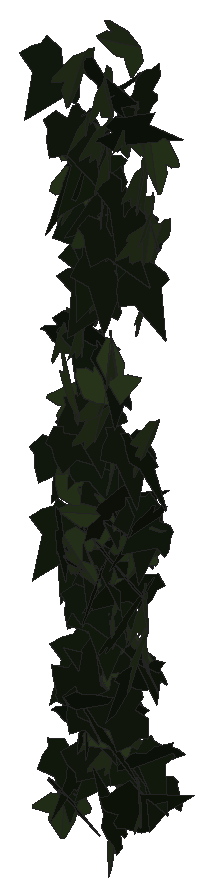
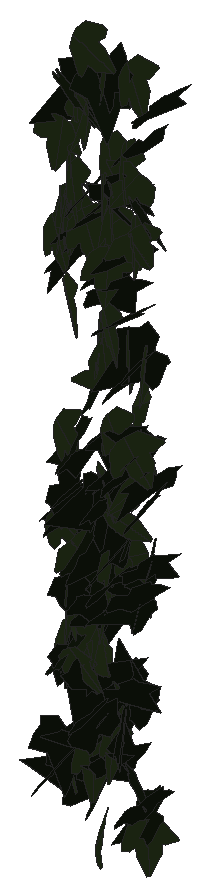
# SketchUp Ruby script. Lengths in inches.
U = 1.inch
M = Sketchup.active_model
def pt(a) = Geom::Point3d.new(a.map { |v| v * U })
def face(e, loops, mat)
  f = e.add_face(loops[0].map { |a| pt(a) })
  loops[1..].each { |l| e.add_face(l.map { |a| pt(a) }).erase! }
  f.material = f.back_material = mat if mat
  f
end
# faces: each face lists its corners as indices into pts; further lists are holes
def faces(e, pts, list, mat = nil) = list.each { |f| face(e, (f[0].is_a?(Array) ? f : [f]).map { |l| l.map { |i| pts[i] } }, mat) }
# xy, xz, yz: faces in a plane at the given z, y or x. An outline is a flat list of corners, or four numbers for a rectangle; further outlines are holes
def ring(l) = l.size == 4 ? [[l[0], l[1]], [l[2], l[1]], [l[2], l[3]], [l[0], l[3]]] : l.each_slice(2).to_a
def flat(e, list, mat, &to3) = list.each { |f| face(e, (f[0].is_a?(Array) ? f : [f]).map { |l| ring(l).map { |u, v| to3.(u, v) } }, mat) }
def xy(e, z, list, mat = nil) = flat(e, list, mat) { |x, y| [x, y, z] }
def xz(e, y, list, mat = nil) = flat(e, list, mat) { |x, z| [x, y, z] }
def yz(e, x, list, mat = nil) = flat(e, list, mat) { |y, z| [x, y, z] }
def lines(e, pts, list) = list.each { |a, b| e.add_line(pt(pts[a]), pt(pts[b])) }
# prism: a flat outline (further loops are holes) pulled along v
def prism(e, loops, v, mat = nil)
  f = face(e, loops, mat); d = Geom::Vector3d.new(v.map { |x| x * U })
  f.pushpull(f.normal.samedirection?(d) ? d.length : -d.length)
end
def box(e, o, s, mat = nil) = prism(e, [[o, [o[0] + s[0], o[1], o[2]], [o[0] + s[0], o[1] + s[1], o[2]], [o[0], o[1] + s[1], o[2]]]], [0, 0, s[2]], mat)
def at(x, y, z, deg = 0) = Geom::Transformation.translation(pt([x, y, z])) * Geom::Transformation.rotation(ORIGIN, Z_AXIS, deg.degrees)
def axes(o, x, y, z) = Geom::Transformation.new([*x, 0, *y, 0, *z, 0, *pt(o).to_a, 1])
def part(name) = M.definitions.add(name)
# library, detail: a bought-in or finely detailed component or shape, given as its bounding box
def library(name, o, s) = part(name).tap { |d| box(d.entities, o, s) }
def detail(e, o, s) = box(e.add_group.entities, o, s)
def put(e, d, t, mat = nil) = e.add_instance(d, t).tap { |i| i.material = mat if mat }
def group(e, t, mat = nil) = e.add_group.tap { |g| g.transformation = t; g.material = mat if mat }.entities
root = M.entities
M.materials.add("efeu1").color = [18, 25, 13]
M.materials.add("efeu2").color = [43, 57, 29]
c1 = part("ivyleaf_9")
p = [[1.54,2.16,1.25],[1.36,2.04,1.19],[-0.21,0.99,0.68],[-0.71,1.11,0.82],[-0.85,0.86,0.67],[-0.8,0.17,0.21],
  [-0.9,-0.01,0.1],[-0.67,-0.16,-0.02],[-0.08,-0.08,-0.05],[-0.03,-0.6,-0.4],[0.65,-0.88,-0.66],[0.83,-0.6,-0.49],
  [1.29,-0.42,-0.43],[1.8125,-0.07,-0.26],[1.21,0.44,0.15]]
faces(c1.entities,p,[[0,1,2,3,4,5,6,7,8,9,10,11,12,13,14]],"efeu1")
c2 = part("ivyleaf_10")
p = [[0,0.5,-0.03],[-0.0625,2.02,-0.43],[-0.19,2.01,-0.46],[-0.54,1.05,-0.29],[-0.52,0.625,-0.18],[-0.83,0.76,-0.28],
  [-1.16,0.64,-0.33],[-1.15,0.33,-0.24],[-0.77,-0.39,0.02],[-0.3,-0.51,0.16],[0.04,-0.48,0.23],[-0.02,2.01,-0.4375],
  [-0.06,2.01,-0.43],[0.04,-0.49,0.23],[0.67,-0.49,0.14],[1.38,0.36,-0.2],[1.375,0.51,-0.24],[0.81,0.65,-0.19],
  [0.62,0.59,-0.15],[0.6,1.09,-0.28],[0.5,1.23,-0.31]]
faces(c2.entities,p,[[0,1,2,3,4,5,6,7,8,9,10],[11,12,0,13,14,15,16,17,18,19,20]],"efeu2")
put(root,c1,axes([542.89,131,239.64],[-0.3779,-0.8089,0.46344],[-0.07293,-0.47288,-0.88486],[0.9294,-0.36601,0.119]))
put(root,c2,axes([543.15,130.99,206.96],[-0.66582,-0.57985,0.08363],[-0.05947,-0.05906,-0.8829],[0.58282,-0.66845,0.00546]))
put(root,c2,axes([543.24,131.94,224.62],[-0.46964,-0.72041,0.42452],[-0.13793,-0.41349,-0.85427],[0.82474,-0.47938,0.09887]))
put(root,c1,axes([542.82,131.93,221.74],[-0.12699,-0.71118,0.61671],[-0.01814,-0.62033,-0.71909],[0.94115,-0.10791,0.06936]))
put(root,c1,axes([543.11,131.42,219.04],[-0.50635,-0.73157,0.28551],[-0.10708,-0.27222,-0.88743],[0.77798,-0.51362,0.06369]))
put(root,c1,axes([542.8,131.78,208.6],[-0.04358,-0.93003,-0.03017],[0.00357,0.03004,-0.93105],[0.93051,-0.04368,0.00216]))
put(root,c2,axes([543.08,131.96,234.19],[0.53623,0.70675,-0.40833],[-0.22326,-0.34294,-0.88675],[-0.78511,0.58024,-0.02673]))
put(root,c1,axes([543.21,130.5625,219.21],[0.54428,-0.26203,-0.88304],[-0.79645,0.38135,-0.60406],[0.46269,0.96466,-0.00106]))
put(root,c1,axes([543.11,132.07,218.12],[-0.41071,-0.80099,0.01291],[-0.00596,-0.01145,-0.90014],[0.80107,-0.41075,-0.00008]))
put(root,c2,axes([543.24,130.78,228.1875],[0.2371,-0.77248,-0.49054],[0.00963,0.50882,-0.79661],[0.91502,0.19481,0.13549]))
put(root,c1,axes([542.89,130.81,222.96],[0.25631,-0.73221,-0.599],[-0.01345,0.61771,-0.76084],[0.94591,0.20718,0.15149]))
put(root,c2,axes([543.45,131.22,234.19],[0.25548,-0.8284,-0.44473],[-0.05712,0.44633,-0.86419],[0.93849,0.25267,0.06846]))
put(root,c1,axes([543.02,130.64,207.7],[0.81346,-0.27877,0.04132],[0.03921,-0.01305,-0.8599],[0.27908,0.8144,0.00037]))
put(root,c1,axes([543.76,131.79,213.49],[-0.66827,-0.54794,0.11511],[-0.07608,-0.08871,-0.86395],[0.5547,-0.67228,0.02018]))
put(root,c1,axes([543.73,131.04,235.24],[-0.79982,0.24945,-0.51189],[0.47089,-0.20653,-0.83641],[-0.32019,-0.92687,0.04861]))
put(root,c2,axes([544.18,130.14,225.47],[-0.27405,0.55462,-0.9475],[-0.55224,0.7744,0.61302],[0.94889,0.61087,0.08313]))
put(root,c1,axes([543.25,130.58,228.39],[0.79583,0.38797,0.34315],[0.32353,0.1189,-0.88476],[-0.40447,0.85846,-0.03254]))
put(root,c1,axes([543.98,130.84,209],[-0.70461,0.24131,-0.4589],[0.41968,-0.18919,-0.74389],[-0.30444,-0.81931,0.03662]))
put(root,c2,axes([543.3,131.49,236.58],[0.75396,0.17984,0.59982],[0.55207,0.25216,-0.76955],[-0.29553,0.92987,0.09268]))
put(root,c1,axes([543.61,131.87,227.56],[-0.02808,-0.90071,0.3593],[0.01235,-0.35976,-0.90088],[0.96965,-0.0215,0.02187]))
put(root,c1,axes([543.73,131.95,223.26],[-0.18829,-0.87979,0.447],[-0.05558,-0.44489,-0.89904],[0.98526,-0.19323,0.03471]))
put(root,c2,axes([543.9375,130.125,222.19],[-0.0737,0.28472,1.03336],[-0.16617,1.02025,-0.29295],[-1.05891,-0.17992,-0.02595]))
put(root,c1,axes([543.26,130.9375,217.57],[0.98692,-0.25548,0.22779],[0.22591,-0.0361,-1.01923],[0.25715,1.01222,0.02114]))
put(root,c2,axes([544.03,131.05,237.25],[0.23393,-0.93139,-0.19948],[0.08891,0.22586,-0.95031],[0.94835,0.20857,0.1383]))
put(root,c2,axes([544.125,130.74,228.55],[0.32713,-0.84864,-0.28411],[0.0021,0.30322,-0.90332],[0.89493,0.3095,0.10597]))
put(root,c1,axes([543.73,130.49,224.01],[0.38574,-0.46473,-0.76294],[-0.14643,0.7869,-0.55336],[0.88126,0.33417,0.24201]))
put(root,c1,axes([543.72,130.51,237.65],[0.33057,-0.8505,-0.42959],[-0.06936,0.43203,-0.90869],[0.95031,0.32738,0.08312]))
put(root,c1,axes([543.9375,131.6,232.93],[-0.14804,-0.95082,-0.18639],[0.03232,0.1836,-0.96227],[0.96838,-0.15148,0.00362]))
put(root,c2,axes([544.27,130.5,240.52],[0.02264,-1.00792,0.16981],[0.02162,-0.16934,-1.00802],[1.0219,0.02591,0.01756]))
put(root,c1,axes([544.13,131.85,229.92],[-0.44896,-0.79228,0.37654],[0.09111,-0.46282,-0.86518],[0.87246,-0.35936,0.28412]))
put(root,c1,axes([543.89,131.62,211.62],[0.0403,-0.11201,-0.9374],[0.79808,-0.49716,0.09371],[-0.50431,-0.79572,0.0734]))
put(root,c2,axes([544.4,131.86,230.02],[0.379,-0.88542,-0.04677],[-0.01625,0.04392,-0.96312],[0.8865,0.37934,0.00234]))
put(root,c1,axes([544.57,131.59,235.91],[-0.80316,-0.57999,0.09291],[-0.08006,-0.04783,-0.99065],[0.5819,-0.8071,-0.00805]))
put(root,c1,axes([544.35,131.87,231.39],[-0.5032,-0.82989,0.02779],[-0.00045,-0.03222,-0.97039],[0.83035,-0.50294,0.01632]))
put(root,c1,axes([544.13,131.45,224.69],[-0.21768,-0.82836,-0.40314],[0.13178,0.38199,-0.85604],[0.91178,-0.25297,0.02747]))
put(root,c1,axes([544.17,132.02,218.18],[-0.14497,-0.949,0.24615],[0.01215,-0.25055,-0.95879],[0.98032,-0.13723,0.04829]))
put(root,c1,axes([543.91,131.52,211.12],[0.14321,-0.23238,-0.90435],[0.84805,-0.35047,0.22435],[-0.39071,-0.84589,0.15549]))
put(root,c2,axes([545.1,130.76,220.5625],[0.31254,0.01615,-0.956],[-0.93757,0.20243,-0.3031],[0.18752,0.98521,0.07795]))
put(root,c2,axes([544.49,131.76,232.7],[-0.53636,-0.82147,-0.06115],[0.08949,0.01443,-0.97878],[0.81887,-0.53964,0.06691]))
put(root,c2,axes([544.5,131.44,225.03],[0.09234,-0.92048,0.18319],[0.01015,-0.18308,-0.92507],[0.93848,0.09255,-0.00802]))
put(root,c1,axes([544.41,130.3,212.39],[-0.74534,0.16412,0.5402],[0.45539,-0.35408,0.73589],[0.33373,0.84969,0.20232]))
put(root,c2,axes([544.63,131.23,210.75],[-0.02239,-0.81588,-0.30481],[0.00737,0.30473,-0.81619],[0.87093,-0.02355,-0.00093]))
put(root,c2,axes([544,130.43,218.94],[-0.51949,0.16153,-0.83821],[0.72315,-0.43811,-0.53261],[-0.45359,-0.88348,0.11086]))
put(root,c2,axes([544.66,131.21,218.7],[-0.08775,-0.87943,-0.25482],[-0.0076,0.25667,-0.88322],[0.91557,-0.08215,-0.03175]))
put(root,c1,axes([544.78,131,209.34],[-0.52719,-0.63291,0.45548],[0.34478,0.30394,0.8214],[-0.6994,0.6269,0.0616]))
put(root,c2,axes([544.75,130.97,224.47],[-0.00558,-0.9292,-0.11369],[-0.03149,0.11381,-0.92867],[0.9356,-0.00171,-0.03193]))
put(root,c1,axes([544.39,131.28,222.88],[0.14621,-0.82186,-0.40667],[0.00957,0.41315,-0.83152],[0.91692,0.12674,0.07352]))
put(root,c2,axes([544.85,131.14,237.3125],[0.13517,-0.99131,-0.1389],[-0.00715,0.1392,-1.00042],[1.00097,0.13486,0.01161]))
put(root,c1,axes([544.45,130.69,212.2],[0.36629,-0.81594,-0.43061],[-0.13641,0.41031,-0.89352],[0.91245,0.38889,0.03928]))
put(root,c1,axes([544.77,132.06,217.47],[-0.32741,-0.90946,-0.21573],[0.04375,0.21342,-0.96612],[0.93367,-0.32892,-0.03038]))
put(root,c1,axes([545.21,131.78,209.6],[-0.64334,-0.61132,0.22429],[-0.1528,-0.16477,-0.88736],[0.63298,-0.6611,0.01376]))
put(root,c1,axes([544.54,129.71,212.3],[0.83497,0.39922,0.37226],[0.32663,0.17967,-0.92529],[-0.43735,0.89637,0.01967]))
put(root,c1,axes([544.62,131.47,218.85],[0.33232,-0.87598,-0.00707],[-0.00069,0.0073,-0.9369],[0.87601,0.33232,0.00195]))
put(root,c2,axes([545.07,131.38,222.36],[0.624,-0.68664,0.00438],[-0.00723,-0.01249,-0.92772],[0.68661,0.62389,-0.01375]))
put(root,c2,axes([545.13,131.06,236.22],[0.3469,-0.84828,-0.3577],[0.02301,0.39012,-0.90286],[0.92033,0.31,0.1574]))
put(root,c1,axes([544.77,131.49,221.6],[0.17194,-0.89909,-0.13673],[-0.04854,0.12988,-0.91509],[0.90813,0.17717,-0.02302]))
put(root,c1,axes([545.71,131.39,212.71],[0.01896,0.05867,0.96721],[-0.96899,0.00306,0.01881],[-0.00192,-0.96739,0.05871]))
put(root,c2,axes([545.12,130.93,234.16],[-0.39132,0.84013,-0.29287],[-0.08317,-0.35309,-0.90174],[-0.88582,-0.33799,0.21405]))
put(root,c1,axes([544.67,130.67,216.97],[-0.15749,-0.47439,-0.79773],[0.46384,0.66062,-0.48443],[0.80392,-0.4741,0.12322]))
put(root,c1,axes([544.96,130.86,219.74],[0.843,0.42216,0.07732],[0.06838,0.03613,-0.9428],[-0.4237,0.84577,0.00168]))
put(root,c1,axes([545.04,132.06,212.09],[-0.06765,-0.88522,0.12997],[0.01522,-0.13146,-0.88745],[0.89458,-0.0647,0.02493]))
put(root,c1,axes([545.5,129.53,217.14],[0.08274,0.21127,0.97971],[0.08019,0.97849,-0.21778],[-0.99902,0.09604,0.06366]))
put(root,c1,axes([545.85,130.86,234.87],[-0.96134,0.16596,0.05366],[-0.05921,-0.0278,-0.97484],[-0.16406,-0.96244,0.03741]))
put(root,c1,axes([545.15,131.23,216.28],[-0.39724,-0.84554,-0.33297],[0.16443,0.29052,-0.9339],[0.89374,-0.42927,0.02382]))
put(root,c1,axes([544.62,131.31,218.57],[0.62656,-0.57058,0.56143],[0.44174,-0.34812,-0.84677],[0.66755,0.76589,0.03338]))
put(root,c1,axes([545.85,130.41,239.56],[-0.0218,0.95328,0.2503],[-0.25104,0.23673,-0.92348],[-0.95309,-0.08416,0.23751]))
put(root,c2,axes([545.54,131.38,210.03],[-0.25674,-1.00139,-0.13294],[0.01344,0.13376,-1.03358],[1.01008,-0.25631,-0.02003]))
put(root,c1,axes([544.68,132.16,211.49],[0.07255,-0.40244,1.01679],[0.73981,-0.73236,-0.34266],[0.8053,0.70907,0.22319]))
put(root,c2,axes([545.16,131.16,213.97],[0.26756,-0.89635,-0.51151],[0.20997,-0.47009,0.9336],[-1.01045,-0.33503,0.05856]))
put(root,c2,axes([545.19,131.05,212.81],[-0.69693,-0.21557,-0.487],[0.52741,-0.16798,-0.68041],[0.07395,-0.83346,0.26309]))
put(root,c1,axes([545.25,130.83,231.6875],[-0.01987,-0.96097,0.02757],[0.00473,-0.02767,-0.96116],[0.96135,-0.01973,0.0053]))
put(root,c2,axes([545.42,130.3,233.65],[-0.65723,-0.58846,-0.40322],[0.34912,0.21278,-0.87959],[0.62209,-0.74112,0.06763]))
put(root,c2,axes([546.2,131.14,241.64],[0.32971,0.14151,-0.93722],[-0.87004,0.4389,-0.23981],[0.37608,0.89132,0.26688]))
put(root,c2,axes([545.23,131.22,216.13],[-0.26887,0.2972,-0.79231],[0.37025,-0.70623,-0.39056],[-0.76092,-0.44866,0.08993]))
put(root,c2,axes([546.03,130.68,211.64],[0.63487,0.02719,-0.70769],[-0.70567,-0.05628,-0.63522],[-0.06003,0.94907,-0.01739]))
put(root,c1,axes([545.08,131.52,226.58],[0.23845,-0.82155,0.67292],[0.14379,-0.65834,-0.85471],[1.05218,0.27616,-0.0357]))
put(root,c2,axes([545.15,131.44,205.92],[0.04444,-0.25729,0.94876],[0.69854,-0.65996,-0.21169],[0.69165,0.68306,0.15284]))
put(root,c2,axes([546.08,131.875,214.14],[-0.73232,0.16904,0.49146],[-0.50826,-0.41029,-0.61623],[0.10855,-0.7807,0.43027]))
put(root,c1,axes([545.49,130.46,220.78],[-0.06861,0.61433,-0.87602],[-0.20028,0.85494,0.61523],[1.05105,0.20301,0.06004]))
put(root,c2,axes([545.56,130.42,226.41],[0.6561,0.74984,-0.18852],[0.12336,0.14256,0.99636],[0.76327,-0.6676,0.00102]))
put(root,c2,axes([545.49,131.58,215.29],[-0.71966,0.53653,-0.33194],[0.26012,-0.20642,-0.89759],[-0.57479,-0.76517,0.00939]))
put(root,c2,axes([545.76,130.08,240.08],[0.24221,-0.85358,-0.45244],[0.0748,0.48161,-0.86857],[0.96317,0.17725,0.18123]))
put(root,c2,axes([545.93,131.33,233.71],[-0.34251,-0.89122,0.22495],[-0.00479,-0.23832,-0.95151],[0.91916,-0.33334,0.07886]))
put(root,c1,axes([545.24,130.36,211.58],[0.81852,-0.6342,0.03381],[0.02998,-0.01651,-1.03545],[0.63439,0.81905,0.0053]))
put(root,c1,axes([545.08,130.7,239.68],[0.25297,-0.35278,0.9231],[0.66556,-0.64352,-0.42833],[0.73047,0.70851,0.07058]))
put(root,c2,axes([546.08,131.76,219.17],[0.34388,0.66767,-0.50509],[-0.32746,-0.39526,-0.74545],[-0.7705,0.46598,0.09139]))
put(root,c1,axes([546.25,130.4,207.02],[0.05635,-0.81228,0.5586],[-0.03098,0.55778,0.8142],[-0.98533,-0.06399,0.00635]))
put(root,c1,axes([546.3125,131.79,217.79],[-0.19713,0.05449,-0.90117],[0.01794,-0.92199,-0.05968],[-0.90264,-0.03023,0.19562]))
put(root,c2,axes([546.1,130.12,228.38],[0.44717,-0.71012,-0.55555],[-0.06305,0.59398,-0.80999],[0.89941,0.3947,0.21943]))
put(root,c1,axes([545.71,131.72,223.625],[0.11371,-0.91598,-0.09853],[-0.0229,0.09643,-0.92295],[0.92098,0.1155,-0.01079]))
put(root,c1,axes([546.83,130.5625,212.54],[-0.26617,-0.26153,-0.9192],[-0.67998,-0.61865,0.37292],[-0.67153,0.73009,-0.01327]))
put(root,c1,axes([545.6,132.2,219.16],[0.18802,-0.66422,0.67362],[0.25573,-0.62555,-0.68819],[0.9108,0.31275,0.05417]))
put(root,c2,axes([546.07,131.49,238.67],[-0.79098,0.56761,-0.16698],[0.1105,-0.13215,-0.97265],[-0.58125,-0.79754,0.04232]))
put(root,c1,axes([545.77,130.12,234.03],[0.47195,-0.77385,-0.56417],[-0.07152,0.59872,-0.88107],[0.955,0.42726,0.21283]))
put(root,c1,axes([546.07,131.85,233.6],[-0.28441,-0.89267,0.27207],[0.06402,-0.30242,-0.92532],[0.93101,-0.2519,0.14674]))
put(root,c2,axes([546.37,131.57,235.72],[0.28843,-0.94608,-0.0449],[0.07262,0.06889,-0.98502],[0.94436,0.28366,0.08946]))
put(root,c1,axes([546.11,131.15,234.79],[-0.00422,-0.88668,0.46932],[0.05356,-0.46885,-0.88532],[1.0018,0.02133,0.04931]))
put(root,c1,axes([546.97,131.46,239.7],[-0.87321,0.46178,-0.11175],[0.07025,-0.10576,-0.98596],[-0.46989,-0.87396,0.06026]))
put(root,c1,axes([546.41,129.74,215.79],[-0.403,0.9419,-0.05473],[-0.02176,0.05022,1.02449],[0.94324,0.40359,0.00025]))
put(root,c2,axes([546.62,131.6,230.47],[0.5011,-0.81653,-0.07831],[-0.02058,0.07922,-0.95773],[0.82002,0.50095,0.02382]))
put(root,c2,axes([546.74,130.59,238.68],[0.23788,-0.94099,-0.26327],[-0.04156,0.26097,-0.97033],[0.97624,0.2404,0.02284]))
put(root,c2,axes([546.77,131.21,216.81],[0.28737,-0.83674,-0.59524],[-0.07236,0.60007,-0.87846],[1.0243,0.27714,0.10493]))
put(root,c1,axes([546.85,131.15,214.08],[-0.1877,0.45805,-0.73656],[0.2237,-0.70256,-0.49391],[-0.83803,-0.29013,0.03314]))
put(root,c2,axes([546.68,131.87,224.32],[0.21344,-0.82322,0.38631],[0.11073,-0.37033,-0.85034],[0.90259,0.2401,0.01297]))
put(root,c1,axes([546.57,131.72,220.47],[-0.03626,-0.92196,0.14939],[-0.01696,-0.14883,-0.92261],[0.93383,-0.0385,-0.01096]))
put(root,c2,axes([547.03,131.37,234.16],[-0.63571,0.65895,0.3624],[-0.28831,0.22473,-0.91436],[-0.69457,-0.69639,0.04785]))
put(root,c1,axes([547.02,131.25,210.3],[0.25234,0.8284,-0.24232],[-0.09411,-0.22455,-0.86566],[-0.85797,0.26828,0.02368]))
put(root,c1,axes([546.32,131.49,223.625],[0.55489,-0.74253,0.11901],[0.07311,-0.09393,-0.92696],[0.74844,0.55968,0.00232]))
put(root,c1,axes([546.43,131.44,210.11],[-0.17307,-0.60211,-0.67608],[0.42173,0.55545,-0.60265],[0.8011,-0.4225,0.1712]))
put(root,c2,axes([547.05,131.37,234.35],[0.38854,-0.84191,-0.32221],[-0.05736,0.32706,-0.92377],[0.89964,0.38447,0.08026]))
put(root,c1,axes([546.45,131.82,214.23],[0.19515,-0.73959,0.47212],[0.2621,-0.41244,-0.75444],[0.83737,0.30146,0.12611]))
put(root,c2,axes([547.03,131.83,233.33],[0.00975,-0.96424,0.1374],[0.05351,-0.13667,-0.96291],[0.97251,0.01719,0.0516]))
put(root,c2,axes([547.06,130.96,236.1],[0.50773,-0.79118,-0.36436],[-0.04451,0.39762,-0.92544],[0.86992,0.48212,0.16531]))
put(root,c2,axes([547.27,130.91,214.61],[-0.59068,0.49166,0.45198],[-0.33161,0.30784,-0.76824],[-0.5797,-0.67707,-0.02108]))
put(root,c2,axes([547.2,131.42,219.92],[-0.1101,-0.73271,0.51048],[-0.08981,-0.50265,-0.74084],[0.88847,-0.1416,-0.01163]))
put(root,c2,axes([547.13,130.71,233.76],[-0.0813,-0.95089,-0.21279],[0.03778,0.21029,-0.95417],[0.97368,-0.08755,0.01926]))
put(root,c2,axes([547.08,130.79,215.47],[0.50452,-0.84163,0.19293],[0.09103,-0.17036,-0.98122],[0.85865,0.51258,-0.00934]))
put(root,c1,axes([546.49,130.3125,207.9375],[0.30701,0.04655,0.93936],[0.91784,0.20083,-0.30992],[-0.20526,0.96764,0.01914]))
put(root,c1,axes([547.35,131.09,221.15],[-0.44555,0.32587,-0.73762],[0.37074,-0.6656,-0.51799],[-0.71612,-0.54733,0.19076]))
put(root,c2,axes([547.23,131.39,237.47],[-0.97782,0.10966,-0.10936],[0.07996,-0.24119,-0.95685],[-0.13263,-0.9539,0.22936]))
put(root,c1,axes([546.78,129.58,238.68],[0.71093,0.48786,0.56603],[0.45142,0.34221,-0.86193],[-0.5955,0.84184,0.02236]))
put(root,c1,axes([547.17,131.69,220.56],[-0.3119,-0.57141,0.66335],[-0.10054,-0.67615,-0.62971],[0.86973,-0.28308,0.1651]))
put(root,c1,axes([546.95,132.32,208.77],[-0.043,-0.80942,0.46465],[0.03439,-0.4662,-0.80894],[0.93267,-0.02012,0.05125]))
put(root,c1,axes([546.93,130.84,231.875],[0.27433,-0.83287,-0.40037],[-0.09104,0.39125,-0.87628],[0.91961,0.28719,0.03268]))
put(root,c2,axes([546.8,130.99,208.25],[-0.00973,0.04122,0.89847],[0.72313,-0.53392,0.03233],[0.53481,0.72268,-0.02736]))
